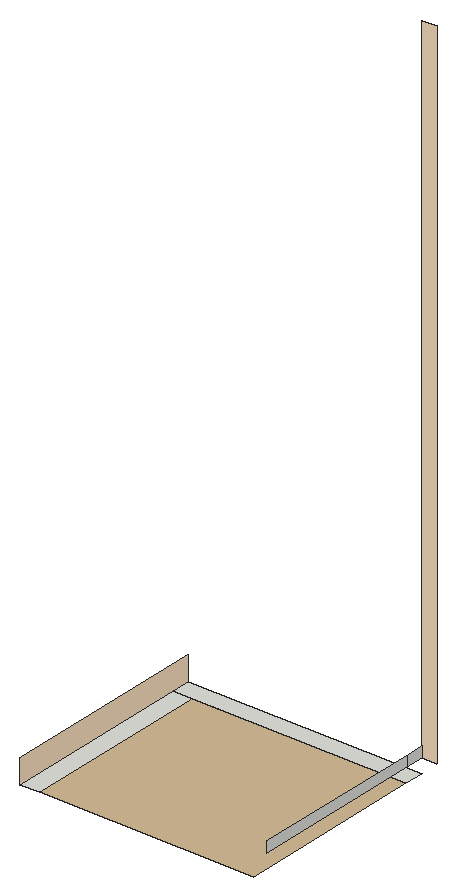
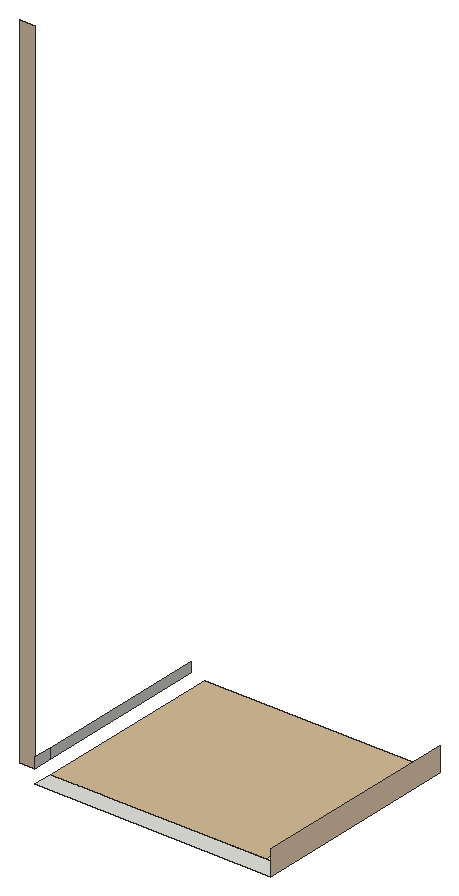
# SketchUp Ruby script. Lengths in inches.
U = 1.inch
M = Sketchup.active_model
def pt(a) = Geom::Point3d.new(a.map { |v| v * U })
def face(e, loops, mat)
  f = e.add_face(loops[0].map { |a| pt(a) })
  loops[1..].each { |l| e.add_face(l.map { |a| pt(a) }).erase! }
  f.material = f.back_material = mat if mat
  f
end
# faces: each face lists its corners as indices into pts; further lists are holes
def faces(e, pts, list, mat = nil) = list.each { |f| face(e, (f[0].is_a?(Array) ? f : [f]).map { |l| l.map { |i| pts[i] } }, mat) }
# xy, xz, yz: faces in a plane at the given z, y or x. An outline is a flat list of corners, or four numbers for a rectangle; further outlines are holes
def ring(l) = l.size == 4 ? [[l[0], l[1]], [l[2], l[1]], [l[2], l[3]], [l[0], l[3]]] : l.each_slice(2).to_a
def flat(e, list, mat, &to3) = list.each { |f| face(e, (f[0].is_a?(Array) ? f : [f]).map { |l| ring(l).map { |u, v| to3.(u, v) } }, mat) }
def xy(e, z, list, mat = nil) = flat(e, list, mat) { |x, y| [x, y, z] }
def xz(e, y, list, mat = nil) = flat(e, list, mat) { |x, z| [x, y, z] }
def yz(e, x, list, mat = nil) = flat(e, list, mat) { |y, z| [x, y, z] }
def lines(e, pts, list) = list.each { |a, b| e.add_line(pt(pts[a]), pt(pts[b])) }
# prism: a flat outline (further loops are holes) pulled along v
def prism(e, loops, v, mat = nil)
  f = face(e, loops, mat); d = Geom::Vector3d.new(v.map { |x| x * U })
  f.pushpull(f.normal.samedirection?(d) ? d.length : -d.length)
end
def box(e, o, s, mat = nil) = prism(e, [[o, [o[0] + s[0], o[1], o[2]], [o[0] + s[0], o[1] + s[1], o[2]], [o[0], o[1] + s[1], o[2]]]], [0, 0, s[2]], mat)
def at(x, y, z, deg = 0) = Geom::Transformation.translation(pt([x, y, z])) * Geom::Transformation.rotation(ORIGIN, Z_AXIS, deg.degrees)
def axes(o, x, y, z) = Geom::Transformation.new([*x, 0, *y, 0, *z, 0, *pt(o).to_a, 1])
def part(name) = M.definitions.add(name)
# library, detail: a bought-in or finely detailed component or shape, given as its bounding box
def library(name, o, s) = part(name).tap { |d| box(d.entities, o, s) }
def detail(e, o, s) = box(e.add_group.entities, o, s)
def put(e, d, t, mat = nil) = e.add_instance(d, t).tap { |i| i.material = mat if mat }
def group(e, t, mat = nil) = e.add_group.tap { |g| g.transformation = t; g.material = mat if mat }.entities
root = M.entities
M.materials.add("[0012_Bisque]3").color = [255, 228, 196]
M.materials.add("[Formica Beige]").color = [211, 187, 149]
xy(root,95.625,[[65.97,364.57,77.31,476.15],[65.97,476.15,202.72,487.49]])
xy(root,95.625,[[77.31,364.57,202.72,476.15]],"[Formica Beige]")
xz(root,487.49,[[202.72,103.6875,211.5,490.375]],"[0012_Bisque]3")
yz(root,65.97,[[364.57,95.625,487.49,109.8125]],"[0012_Bisque]3")
yz(root,202.72,[[374.1875,103.6875,476.36,109.8125],[476.36,103.6875,487.49,109.8125]])
